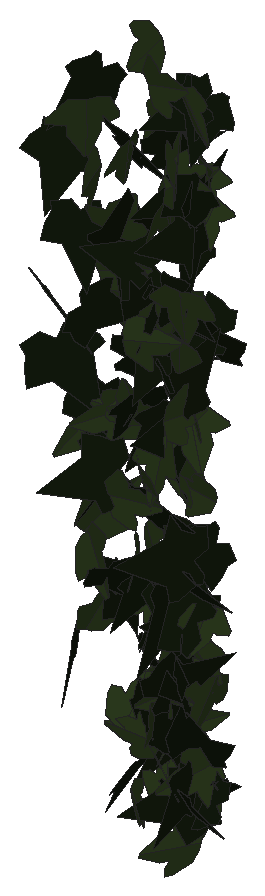
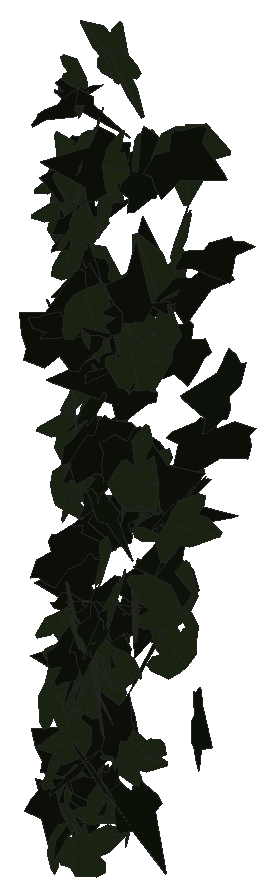
# SketchUp Ruby script. Lengths in inches.
U = 1.inch
M = Sketchup.active_model
def pt(a) = Geom::Point3d.new(a.map { |v| v * U })
def face(e, loops, mat)
  f = e.add_face(loops[0].map { |a| pt(a) })
  loops[1..].each { |l| e.add_face(l.map { |a| pt(a) }).erase! }
  f.material = f.back_material = mat if mat
  f
end
# faces: each face lists its corners as indices into pts; further lists are holes
def faces(e, pts, list, mat = nil) = list.each { |f| face(e, (f[0].is_a?(Array) ? f : [f]).map { |l| l.map { |i| pts[i] } }, mat) }
# xy, xz, yz: faces in a plane at the given z, y or x. An outline is a flat list of corners, or four numbers for a rectangle; further outlines are holes
def ring(l) = l.size == 4 ? [[l[0], l[1]], [l[2], l[1]], [l[2], l[3]], [l[0], l[3]]] : l.each_slice(2).to_a
def flat(e, list, mat, &to3) = list.each { |f| face(e, (f[0].is_a?(Array) ? f : [f]).map { |l| ring(l).map { |u, v| to3.(u, v) } }, mat) }
def xy(e, z, list, mat = nil) = flat(e, list, mat) { |x, y| [x, y, z] }
def xz(e, y, list, mat = nil) = flat(e, list, mat) { |x, z| [x, y, z] }
def yz(e, x, list, mat = nil) = flat(e, list, mat) { |y, z| [x, y, z] }
def lines(e, pts, list) = list.each { |a, b| e.add_line(pt(pts[a]), pt(pts[b])) }
# prism: a flat outline (further loops are holes) pulled along v
def prism(e, loops, v, mat = nil)
  f = face(e, loops, mat); d = Geom::Vector3d.new(v.map { |x| x * U })
  f.pushpull(f.normal.samedirection?(d) ? d.length : -d.length)
end
def box(e, o, s, mat = nil) = prism(e, [[o, [o[0] + s[0], o[1], o[2]], [o[0] + s[0], o[1] + s[1], o[2]], [o[0], o[1] + s[1], o[2]]]], [0, 0, s[2]], mat)
def at(x, y, z, deg = 0) = Geom::Transformation.translation(pt([x, y, z])) * Geom::Transformation.rotation(ORIGIN, Z_AXIS, deg.degrees)
def axes(o, x, y, z) = Geom::Transformation.new([*x, 0, *y, 0, *z, 0, *pt(o).to_a, 1])
def part(name) = M.definitions.add(name)
# library, detail: a bought-in or finely detailed component or shape, given as its bounding box
def library(name, o, s) = part(name).tap { |d| box(d.entities, o, s) }
def detail(e, o, s) = box(e.add_group.entities, o, s)
def put(e, d, t, mat = nil) = e.add_instance(d, t).tap { |i| i.material = mat if mat }
def group(e, t, mat = nil) = e.add_group.tap { |g| g.transformation = t; g.material = mat if mat }.entities
root = M.entities
M.materials.add("efeu1").color = [18, 25, 13]
M.materials.add("efeu2").color = [43, 57, 29]
c1 = part("ivyleaf_9")
p = [[1.54,2.16,1.25],[1.36,2.04,1.19],[-0.21,0.99,0.68],[-0.71,1.11,0.82],[-0.85,0.86,0.67],[-0.8,0.17,0.21],
  [-0.9,-0.01,0.1],[-0.67,-0.16,-0.02],[-0.08,-0.08,-0.05],[-0.03,-0.6,-0.4],[0.65,-0.88,-0.66],[0.83,-0.6,-0.49],
  [1.29,-0.42,-0.43],[1.8125,-0.07,-0.26],[1.21,0.44,0.15]]
faces(c1.entities,p,[[0,1,2,3,4,5,6,7,8,9,10,11,12,13,14]],"efeu1")
c2 = part("ivyleaf_10")
p = [[0,0.5,-0.03],[-0.0625,2.02,-0.43],[-0.19,2.01,-0.46],[-0.54,1.05,-0.29],[-0.52,0.625,-0.18],[-0.83,0.76,-0.28],
  [-1.16,0.64,-0.33],[-1.15,0.33,-0.24],[-0.77,-0.39,0.02],[-0.3,-0.51,0.16],[0.04,-0.48,0.23],[-0.02,2.01,-0.4375],
  [-0.06,2.01,-0.43],[0.04,-0.49,0.23],[0.67,-0.49,0.14],[1.38,0.36,-0.2],[1.375,0.51,-0.24],[0.81,0.65,-0.19],
  [0.62,0.59,-0.15],[0.6,1.09,-0.28],[0.5,1.23,-0.31]]
faces(c2.entities,p,[[0,1,2,3,4,5,6,7,8,9,10],[11,12,0,13,14,15,16,17,18,19,20]],"efeu2")
put(root,c1,axes([577.84,127.46,235.97],[-0.54713,-0.95922,-0.06143],[0.03475,0.0509,-1.10428],[0.96056,-0.54821,0.00496]))
put(root,c1,axes([577.5,126.54,229.15],[0.77126,-0.74947,0.54507],[0.38376,-0.38718,-1.07539],[0.84352,0.86141,-0.00912]))
put(root,c1,axes([578.28,126.27,227.13],[-0.07433,-0.79998,-0.96205],[0.25261,0.93431,-0.79643],[1.22544,-0.24112,0.10582]))
put(root,c2,axes([578.99,127.875,223.36],[0.28958,0.60326,-1.04086],[-0.47539,-0.92608,-0.669],[-1.10513,0.55644,0.01504]))
put(root,c1,axes([579.53,127.46,239.9],[-0.04117,0.14297,-1.10614],[0.26534,-1.07385,-0.14867],[-1.08331,-0.26846,0.00562]))
put(root,c1,axes([578.98,127.55,224.3],[0.19604,-1.04949,-0.00303],[0.00133,0.00333,-1.06764],[1.0495,0.19603,0.00192]))
put(root,c1,axes([579.17,126.42,213.89],[-0.39771,0.17693,-1.07008],[0.95652,-0.4801,-0.43488],[-0.51132,-1.03574,0.01878]))
put(root,c1,axes([579.46,126.28,233.58],[-0.18909,-1.0455,-0.36243],[0.03266,0.36225,-1.06202],[1.10606,-0.18943,-0.03061]))
put(root,c1,axes([580.44,127.05,224.01],[0.07064,-0.08019,1.08996],[-0.81245,0.72671,0.10612],[-0.73102,-0.81541,-0.01261]))
put(root,c2,axes([579.57,127.04,235.33],[-0.19467,0.12924,1.16872],[0.74273,-0.90487,0.22378],[0.91157,0.76487,0.06726]))
put(root,c1,axes([579.52,127.14,222.07],[0.68191,-0.83193,-0.06586],[-0.03563,0.05594,-1.07566],[0.83377,0.6828,0.00789]))
put(root,c2,axes([579.84,126.89,218.9375],[-0.21285,-0.85941,0.88653],[0.20724,0.86198,0.88537],[-1.2172,0.29704,-0.00429]))
put(root,c2,axes([580.36,125.55,239.22],[-0.77769,-0.98029,0.00301],[-0.00247,-0.00188,-1.25131],[0.98029,-0.7777,-0.00076]))
put(root,c1,axes([580.32,125.96,220.41],[-0.48808,0.83569,-0.60486],[-0.30344,0.52324,0.96778],[0.98598,0.57471,-0.00157]))
put(root,c2,axes([580.78,127.27,224.34],[0.06351,0.07636,-1.12488],[-0.68801,-0.88995,-0.09926],[-0.89321,0.69093,-0.00353]))
put(root,c1,axes([580.45,125.3,230],[0.12902,0.0871,-1.06262],[-0.28217,1.03499,0.05058],[1.02817,0.27311,0.14723]))
put(root,c1,axes([581.4,126.1,222.16],[-0.76216,-0.34163,0.78875],[-0.68327,-0.39879,-0.83296],[0.52152,-1.02175,0.06139]))
put(root,c2,axes([580.21,125.89,218.39],[0.6743,-0.13921,1.01089],[0.98144,-0.24326,-0.68816],[0.27938,1.19055,-0.02241]))
put(root,c2,axes([580.72,127,233.17],[-0.8731,-0.50427,0.41981],[0.41244,0.12171,1.00395],[-0.51032,0.96111,0.09313]))
put(root,c2,axes([580.31,127.05,230.83],[-0.35512,-0.21894,0.97012],[0.9139,0.33446,0.41002],[-0.39226,0.97744,0.07701]))
put(root,c2,axes([581.5,127.78,223.99],[0.25173,0.45175,0.97861],[-0.5041,-0.83892,0.51693],[0.9527,-0.56326,0.01495]))
put(root,c1,axes([580.76,127.23,232.55],[0.7363,0.68159,0.59625],[-0.44424,-0.39779,1.00331],[0.78913,-0.85989,0.00848]))
put(root,c2,axes([581.02,125.22,215.46],[-0.10064,-0.95278,0.44517],[0.04897,0.44247,0.95808],[-1.05051,0.11191,0.00201]))
put(root,c2,axes([581.26,127.53,229.1875],[-0.99481,-0.40426,0.26465],[0.26705,0.04482,1.07228],[-0.40268,1.02843,0.0573]))
put(root,c1,axes([580.97,127.16,216.3],[0.58161,-0.472,-0.92215],[0.70238,-0.59767,0.74892],[-0.76145,-0.91182,-0.01354]))
put(root,c2,axes([581.79,127.14,224.44],[-0.9632,-0.14803,-0.23744],[-0.22743,-0.08157,0.97348],[-0.16298,0.98867,0.04477]))
put(root,c1,axes([582.13,127.58,231.55],[-0.35685,-0.77533,-0.61729],[-0.2258,-0.57522,0.85303],[-0.96498,0.42132,0.02867]))
put(root,c1,axes([582.1,127.01,225.5],[-0.14828,0.8337,-0.54836],[-0.00473,-0.55496,-0.84246],[-0.99786,-0.12126,0.08548]))
put(root,c2,axes([582.66,126.71,229.09],[-0.10819,0.17491,1.03635],[-1.04823,0.05779,-0.11918],[-0.07641,-1.04038,0.16761]))
put(root,c1,axes([582.1,124.95,218.28],[0.6077,0.86851,-0.0681],[-0.04334,-0.05278,-1.05999],[-0.8701,0.60922,0.00524]))
put(root,c2,axes([582.41,126.25,218.46],[0.35652,-0.67819,-0.65364],[-0.2456,0.60779,-0.76457],[0.90932,0.43006,0.04977]))
put(root,c1,axes([582.6875,125.99,208.91],[-0.53228,0.9446,-0.37856],[0.18281,-0.33151,-1.08424],[-1.00108,-0.56279,0.00329]))
put(root,c1,axes([581.4,126.44,237.77],[0.83554,-0.52381,0.63201],[0.54256,-0.32434,-0.98609],[0.61599,0.99618,0.01127]))
put(root,c2,axes([582.78,126.86,242.56],[0.81683,-0.44863,-0.67769],[-0.58594,0.34076,-0.93183],[0.56321,1.00517,0.01343]))
put(root,c2,axes([582.1,128.14,238.61],[0.22968,-0.50762,0.92929],[0.47351,-0.80129,-0.55474],[0.94712,0.5237,0.05198]))
put(root,c2,axes([582.57,125.42,238.1875],[0.09223,-0.99717,-0.22009],[-0.01567,0.21957,-1.00142],[1.02105,0.09344,0.00451]))
put(root,c2,axes([582.42,127.22,219.07],[-0.34586,0.90517,0.03982],[-0.00834,0.03943,-0.96897],[-0.90601,-0.3459,-0.00628]))
put(root,c1,axes([583.24,125.55,229.87],[-0.13012,0.25225,1.18893],[-0.61048,1.02037,-0.2833],[-1.05095,-0.62395,0.01737]))
put(root,c2,axes([582.28,125.9375,210.99],[0.92914,0.36434,-0.45422],[0.29752,0.43823,0.9601],[0.50054,-0.93679,0.27248]))
put(root,c1,axes([581.9375,127.8,212.6],[0.16746,-0.32979,0.92983],[0.46743,-0.80404,-0.36936],[0.86883,0.49614,0.0195]))
put(root,c2,axes([582.33,127.43,216.03],[0.92597,0.0672,0.25461],[0.25418,0.01509,-0.9284],[-0.0688,0.96022,-0.00322]))
put(root,c2,axes([583.43,125.77,210.41],[0.13143,0.08378,0.99588],[-0.93124,-0.35433,0.15271],[0.36276,-0.93995,0.03119]))
put(root,c1,axes([583.34,127.18,222.6],[-0.61025,0.67861,-0.01763],[0.00879,-0.0158,-0.91264],[-0.67878,-0.6103,0.00402]))
put(root,c1,axes([583.07,126.16,217.55],[-0.08693,0.3958,-0.81261],[0.17359,-0.79385,-0.40524],[-0.88705,-0.19414,0.00033]))
put(root,c2,axes([582.1,125.46,221.41],[-0.17856,-0.08973,1.07178],[1.03727,0.27282,0.19565],[-0.2843,1.05174,0.04068]))
put(root,c1,axes([583.58,125.81,215.85],[-0.46194,0.29027,-0.79342],[-0.67142,0.42274,0.54556],[0.5128,0.81498,-0.0004]))
put(root,c1,axes([582.32,125.95,228.04],[0.7614,0.17439,1.00684],[0.97914,0.23464,-0.78109],[-0.29228,1.24033,0.0062]))
put(root,c2,axes([583.375,125.55,222.96],[-0.82796,0.54206,0.17614],[-0.15701,0.0817,-0.98947],[-0.54791,-0.84253,0.01738]))
put(root,c2,axes([583.41,124.98,207.98],[-0.44007,0.69425,0.35046],[-0.23702,0.26379,-0.82018],[-0.74069,-0.49688,0.05424]))
put(root,c1,axes([583.28,126.96,228.54],[-0.43551,-0.89185,0.20402],[-0.09226,-0.18199,-0.9925],[0.91022,-0.44517,-0.00298]))
put(root,c1,axes([583.71,127.04,225.24],[-0.01678,0.49688,-0.9755],[-0.00978,-0.97564,-0.49679],[-1.09471,0.0011,0.01939]))
put(root,c2,axes([583.27,126.99,220.0625],[-0.50558,0.69346,-0.28764],[0.17448,-0.22875,-0.85818],[-0.73019,-0.53481,-0.0059]))
put(root,c1,axes([584.14,127.36,210.79],[-1.20845,0.48774,-0.275],[0.25514,-0.10262,-1.30317],[-0.49842,-1.23509,-0.00032]))
put(root,c1,axes([583.55,127.51,216.07],[0.52872,-0.69595,-0.05207],[0.04827,-0.0287,0.87375],[-0.69622,-0.53051,0.02104]))
put(root,c1,axes([583.15,126.79,237.55],[0.30615,0.15951,0.94698],[0.85533,0.4066,-0.34501],[-0.4366,0.90839,-0.01186]))
put(root,c1,axes([583.03,126.02,221.22],[0.58187,-0.26207,0.67929],[0.60039,-0.31921,-0.63744],[0.41188,0.83553,-0.03047]))
put(root,c1,axes([583.42,127.03,227.42],[0.73275,-0.58998,-0.16727],[-0.12651,0.10959,-0.94073],[0.60004,0.74357,0.00593]))
put(root,c2,axes([583.86,128.14,234.76],[-0.01241,0.22249,-1.09936],[-0.15218,-1.0896,-0.2188],[-1.11128,0.14673,0.04224]))
put(root,c2,axes([583.8,126.48,207.84],[0.70447,0.51969,-0.08923],[0.06279,0.06517,0.87529],[0.52355,-0.7071,0.01509]))
put(root,c1,axes([583.31,127.36,223.03],[0.3375,-0.66584,0.52612],[0.26863,-0.45326,-0.74595],[0.80497,0.43042,0.02835]))
put(root,c2,axes([583.11,125.37,229.36],[0.13365,-0.01338,-1.0253],[1.02437,-0.04416,0.13411],[-0.04552,-1.03303,0.00755]))
put(root,c2,axes([583.46,127.15,213.93],[0.73822,-0.5197,0.78557],[0.61092,-0.49551,-0.9019],[0.71693,0.95737,-0.04036]))
put(root,c2,axes([583.875,125.82,211.43],[0.05773,-0.70058,-0.66592],[0.10262,-0.6589,0.70209],[-0.96111,-0.11243,0.03497]))
put(root,c1,axes([583.45,125.67,211.13],[-0.11424,0.14574,1.08683],[0.67522,-0.85163,0.18517],[0.86401,0.68481,-0.00101]))
put(root,c1,axes([584.28,127.65,224.32],[-0.2237,-0.37521,1.22313],[-0.6305,-1.0481,-0.43683],[1.11324,-0.669,-0.00163]))
put(root,c2,axes([584.35,126.73,230.93],[-0.49081,-1.09543,0.24458],[-0.08741,-0.22883,-1.20028],[1.11899,-0.49835,0.01352]))
put(root,c2,axes([584.01,125.73,224.25],[1.13792,-0.38672,0.09151],[0.09216,-0.01319,-1.20171],[0.38656,1.14151,0.01712]))
put(root,c1,axes([583.65,126.44,208.72],[0.26011,-0.46518,0.68463],[0.31978,-0.60545,-0.53287],[0.76345,0.41209,-0.01006]))
put(root,c1,axes([584.01,126.92,216.99],[-0.08696,0.10283,-1.40835],[0.93237,-1.05553,-0.13464],[-1.06053,-0.93641,-0.00289]))
put(root,c2,axes([584.4,125.55,235.99],[0.14126,-0.89008,-0.58968],[-0.03598,0.59051,-0.89996],[1.06709,0.13774,0.04772]))
put(root,c1,axes([584.54,126.66,216.99],[-0.80908,-0.40204,0.02181],[-0.01636,-0.0161,-0.90343],[0.4023,-0.80921,0.00713]))
put(root,c1,axes([584.6,127.96,215.09],[-0.17106,-0.21146,1.18058],[-0.76103,-0.90258,-0.27193],[0.927,-0.78,-0.00539]))
put(root,c1,axes([585.14,127.07,240.4],[-0.9621,0.14444,0.342],[-0.33972,0.04059,-0.97283],[-0.14972,-1.02027,0.00972]))
put(root,c1,axes([585.37,126.34,216.39],[-0.88804,-0.54252,-0.59103],[-0.50816,-0.30187,1.04063],[-0.62082,1.02313,-0.00636]))
put(root,c2,axes([583.73,125.87,212.84],[-0.01968,-0.01757,0.96237],[0.93674,0.22098,0.02319],[-0.22132,0.93686,0.01258]))
put(root,c2,axes([584.82,126.1,213.08],[0.03874,0.11187,-1.05003],[-0.55477,-0.8919,-0.11549],[-0.89851,0.55551,0.02604]))
put(root,c2,axes([584.09,127.66,216.3125],[0.57664,-0.73823,-0.58995],[0.36537,-0.4632,0.93675],[-0.87152,-0.68264,0.00237]))
put(root,c2,axes([584.84,126.23,229.15],[-0.91501,0.00706,0.25488],[-0.25487,0.00325,-0.91503],[-0.00767,-0.94984,-0.00123]))
put(root,c2,axes([584.4375,126.07,212.62],[0.8916,0.59533,-0.18716],[0.15191,0.10953,1.07207],[0.60528,-0.90443,0.00664]))
put(root,c2,axes([585.0625,125.38,237.7],[-0.11332,0.36899,-1.10131],[-0.33556,1.04895,0.38598],[1.11195,0.35416,0.00424]))
put(root,c2,axes([584.85,126.57,222.88],[-0.13975,0.52256,0.78714],[-0.33961,0.71474,-0.5348],[-0.88166,-0.35815,0.08123]))
put(root,c2,axes([584.59,126.92,236.36],[-0.56002,0.79122,-0.12785],[0.08204,-0.09856,-0.9693],[-0.79727,-0.56591,-0.00994]))
put(root,c2,axes([584.1,125.38,241.625],[-0.4177,0.00353,1.01164],[1.01163,0.00762,0.41766],[-0.0057,1.09446,-0.00617]))
put(root,c2,axes([585,126.34,205.7],[-0.03505,0.20769,1.14464],[-0.0556,-1.14415,0.2059],[1.162,-0.04848,0.04437]))
put(root,c1,axes([585.15,127.14,234.13],[-0.41838,-0.40932,1.02251],[-0.61949,-0.81692,-0.5805],[0.91066,-0.74378,0.07487]))
put(root,c2,axes([584.78,126.34,236.85],[-0.94358,-0.15368,-0.24318],[0.24424,0.01264,-0.95566],[0.152,-0.97433,0.02596]))
put(root,c1,axes([585.48,126.52,207.99],[-0.22039,-0.35532,-1.08316],[-0.30216,-1.04555,0.40447],[-1.09918,0.35866,0.10599]))
put(root,c1,axes([585.35,126.2,219.3125],[-0.36284,-0.35594,1.1389],[-0.86963,-0.73619,-0.50713],[0.81701,-0.94168,-0.03401]))
put(root,c1,axes([584.16,125.9,231.79],[0.00159,-0.04771,-1.02887],[0.84004,0.5954,-0.02631],[0.59598,-0.83909,0.03983]))
put(root,c1,axes([584.74,127.71,209.71],[-0.24028,-0.71702,0.51834],[-0.02499,-0.5314,-0.74667],[0.8844,-0.20982,0.11973]))
put(root,c2,axes([585.6,126.76,222.16],[-0.30541,0.05998,-0.88764],[-0.88894,0.01732,0.30702],[0.03592,0.93855,0.05106]))
put(root,c1,axes([585.6875,127.53,229.58],[-0.53006,0.1458,0.80818],[-0.82046,-0.05238,-0.52867],[-0.03555,-0.96508,0.15079]))
put(root,c1,axes([584.67,127.08,234.49],[-0.74933,-0.04783,-1.02163],[1.02274,-0.02929,-0.74878],[0.00465,-1.26664,0.05589]))
put(root,c2,axes([585.53,126.3,226.22],[-0.36366,0.34664,0.87096],[-0.75069,0.45182,-0.49326],[-0.56143,-0.82866,0.09539]))
put(root,c2,axes([584.8,126.78,210.98],[-0.05627,-0.11888,0.8671],[0.19019,0.84647,0.12839],[-0.8543,0.19627,-0.02853]))
put(root,c2,axes([584.78,126.85,225.42],[0.69206,0.83972,0.21674],[0.14083,0.16479,-1.08815],[-0.85573,0.70623,-0.0038]))
put(root,c2,axes([584.93,127.31,236.75],[0.3955,0.88364,0.04265],[0.02362,0.03615,-0.96809],[-0.88436,0.39615,-0.00679]))
put(root,c1,axes([585.63,126.07,236.9375],[-0.21307,0.08696,-0.99059],[-0.23433,-0.98893,-0.03641],[-0.96639,0.22063,0.22723]))
put(root,c2,axes([585.05,127.85,206.77],[0.07316,-0.70069,0.55548],[0.20454,-0.52945,-0.69479],[0.87045,0.1833,0.11657]))
put(root,c2,axes([584.55,127.6875,237.3],[-0.50422,-0.1011,0.93447],[0.88574,-0.40592,0.43402],[0.31449,0.98117,0.27584]))
put(root,c1,axes([584.875,126.41,213.66],[-0.08064,-0.41252,1.14151],[-0.09614,-1.13826,-0.41814],[1.20995,-0.11794,0.04286]))
put(root,c1,axes([584.95,127.83,240.3],[-0.26458,-1.03179,0.19823],[0.03749,-0.21356,-1.06154],[1.04999,-0.25237,0.08785]))
put(root,c1,axes([584.49,125.84,208.21],[0.94157,-0.2457,0.27985],[0.27013,-0.07318,-0.9731],[0.25635,0.97955,-0.0025]))
put(root,c2,axes([584.93,125.625,237.23],[0.03803,-0.09671,-1.09684],[0.47455,0.99178,-0.07099],[0.99359,-0.46998,0.07589]))
put(root,c2,axes([584.97,127.32,235.27],[0.62454,0.7199,0.12917],[0.08185,0.1,-0.95304],[-0.7268,0.62987,0.00367]))
put(root,c2,axes([585.21,126.35,214.02],[0.30757,0.81199,-0.57165],[-0.19671,-0.53676,-0.86827],[-0.97335,0.36506,-0.00516]))
put(root,c1,axes([585.35,125.61,215.03],[0.35573,-0.24734,-0.89616],[-0.71757,0.53702,-0.43306],[0.59109,0.80079,0.01362]))
put(root,c2,axes([585.31,125.14,226.4375],[-0.03827,0.1567,1.04866],[-0.24083,1.02063,-0.1613],[-1.03259,-0.24384,-0.00124]))
put(root,c1,axes([585.21,127.45,228.86],[1.12659,-0.25981,0.56554],[-0.55153,0.1251,1.15616],[-0.28836,-1.25434,-0.00183]))
put(root,c2,axes([585.53,125.42,232.03],[-1.14191,-0.24607,0.11644],[-0.12187,0.01308,-1.16749],[0.24343,-1.14775,-0.03827]))
put(root,c1,axes([585.17,126.52,209.91],[1.02371,0.06123,0.56027],[-0.56145,0.00926,1.02486],[0.04925,-1.16697,0.03753]))
put(root,c2,axes([585.86,126.97,207.96],[0.29829,-0.13468,-0.82812],[-0.72338,0.40394,-0.32626],[0.42501,0.78204,0.02591]))
put(root,c1,axes([585.33,126.35,235.86],[0.02204,0.00237,1.03676],[0.40501,0.95457,-0.01079],[-0.95438,0.40515,0.01936]))
put(root,c1,axes([584.58,126.4375,218.02],[0.66806,-0.32125,0.53796],[0.51125,-0.17516,-0.73949],[0.36225,0.83965,0.05155]))
put(root,c2,axes([585.74,126.77,209.38],[0.26215,0.27278,-1.08927],[-0.71402,-0.82281,-0.37789],[-0.86666,0.7604,-0.01815]))
put(root,c2,axes([585.1,126.98,214.73],[-0.76411,-0.02521,-0.41912],[0.4198,-0.02908,-0.7636],[0.0081,-0.87102,0.03762]))
put(root,c1,axes([586.14,126.6875,207.86],[-0.50656,0.14342,0.77858],[-0.74512,0.22597,-0.52641],[-0.26752,-0.90096,-0.00809]))
put(root,c1,axes([585.5625,127.4,219.61],[0.0055,-0.29628,-1.03574],[0.22718,-1.01215,0.29074],[-1.05306,-0.2199,0.05731]))
put(root,c1,axes([585.5625,126.93,208.16],[0.28705,0.80617,-0.1133],[-0.04446,-0.10443,-0.85573],[-0.81288,0.2904,0.00679]))
put(root,c1,axes([585.11,126.04,227.15],[-0.61117,0.69742,0.82019],[0.51344,-0.64017,0.92693],[0.9463,0.79776,0.02679]))
put(root,c2,axes([585.49,126.93,216.4375],[0.54334,0.64435,-0.34865],[-0.21082,-0.2782,-0.84268],[-0.70164,0.58256,-0.01678]))
put(root,c1,axes([584.99,124.69,213.53],[0.22599,0.19051,1.17744],[0.95242,0.6926,-0.29486],[-0.71803,0.97865,-0.02054]))
put(root,c1,axes([585.38,126.15,208.94],[-0.12476,0.0957,-1.11275],[0.67655,-0.88438,-0.15191],[-0.88862,-0.68676,0.04057]))
put(root,c2,axes([585.07,126.48,240.79],[-0.57706,0.3433,-0.75448],[0.57969,-0.48996,-0.66632],[-0.59249,-0.81374,0.0829]))
put(root,c2,axes([585.69,127.03,213.08],[-0.15007,-1.14491,0.34896],[-0.01335,-0.35007,-1.15429],[1.19684,-0.14746,0.03088]))
